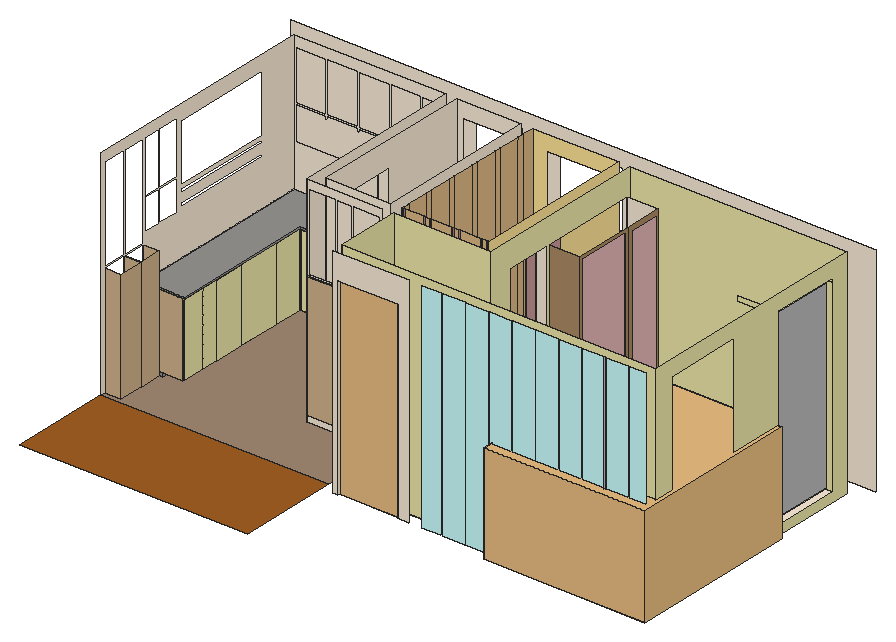
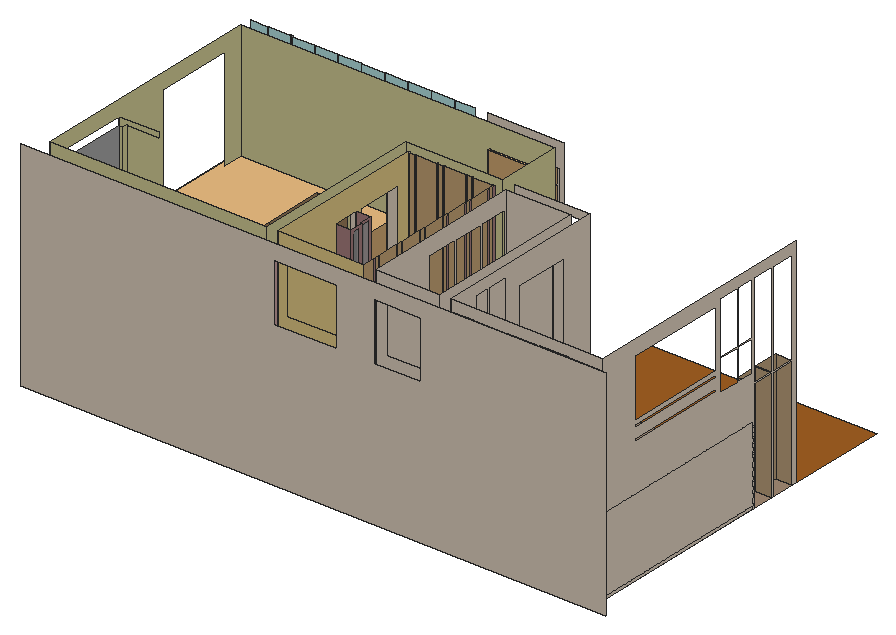
# SketchUp Ruby script. Lengths in inches.
U = 1.inch
M = Sketchup.active_model
def pt(a) = Geom::Point3d.new(a.map { |v| v * U })
def face(e, loops, mat)
  f = e.add_face(loops[0].map { |a| pt(a) })
  loops[1..].each { |l| e.add_face(l.map { |a| pt(a) }).erase! }
  f.material = f.back_material = mat if mat
  f
end
# faces: each face lists its corners as indices into pts; further lists are holes
def faces(e, pts, list, mat = nil) = list.each { |f| face(e, (f[0].is_a?(Array) ? f : [f]).map { |l| l.map { |i| pts[i] } }, mat) }
# xy, xz, yz: faces in a plane at the given z, y or x. An outline is a flat list of corners, or four numbers for a rectangle; further outlines are holes
def ring(l) = l.size == 4 ? [[l[0], l[1]], [l[2], l[1]], [l[2], l[3]], [l[0], l[3]]] : l.each_slice(2).to_a
def flat(e, list, mat, &to3) = list.each { |f| face(e, (f[0].is_a?(Array) ? f : [f]).map { |l| ring(l).map { |u, v| to3.(u, v) } }, mat) }
def xy(e, z, list, mat = nil) = flat(e, list, mat) { |x, y| [x, y, z] }
def xz(e, y, list, mat = nil) = flat(e, list, mat) { |x, z| [x, y, z] }
def yz(e, x, list, mat = nil) = flat(e, list, mat) { |y, z| [x, y, z] }
def lines(e, pts, list) = list.each { |a, b| e.add_line(pt(pts[a]), pt(pts[b])) }
# prism: a flat outline (further loops are holes) pulled along v
def prism(e, loops, v, mat = nil)
  f = face(e, loops, mat); d = Geom::Vector3d.new(v.map { |x| x * U })
  f.pushpull(f.normal.samedirection?(d) ? d.length : -d.length)
end
def box(e, o, s, mat = nil) = prism(e, [[o, [o[0] + s[0], o[1], o[2]], [o[0] + s[0], o[1] + s[1], o[2]], [o[0], o[1] + s[1], o[2]]]], [0, 0, s[2]], mat)
def at(x, y, z, deg = 0) = Geom::Transformation.translation(pt([x, y, z])) * Geom::Transformation.rotation(ORIGIN, Z_AXIS, deg.degrees)
def axes(o, x, y, z) = Geom::Transformation.new([*x, 0, *y, 0, *z, 0, *pt(o).to_a, 1])
def part(name) = M.definitions.add(name)
# library, detail: a bought-in or finely detailed component or shape, given as its bounding box
def library(name, o, s) = part(name).tap { |d| box(d.entities, o, s) }
def detail(e, o, s) = box(e.add_group.entities, o, s)
def put(e, d, t, mat = nil) = e.add_instance(d, t).tap { |i| i.material = mat if mat }
def group(e, t, mat = nil) = e.add_group.tap { |g| g.transformation = t; g.material = mat if mat }.entities
root = M.entities
M.materials.add("Maquette Wood B01 12cm").color = [172, 139, 100]
M.materials.add("Plywood A 50cm\#1").color = [191, 159, 129]
M.materials.add("[0028_AntiqueWhite]").color = [250, 235, 215]
M.materials.add("[0035_Tan]").color = [210, 180, 140]
M.materials.add("[0048_PaleGoldenrod]").color = [238, 232, 170]
M.materials.add("[0119_RosyBrown]").color = [188, 143, 143]
M.materials.add("[0132_LightGray]").color = [169, 169, 169]
M.materials.add("[0134_DimGray]").color = [105, 105, 105]
M.materials.add("[Color D02]").color = [255, 229, 153]
M.materials.add("[Color H01]").color = [204, 255, 255]
M.materials.add("[Color M02]").color = [198, 198, 198]
M.materials.add("[Granite Light Gray]").color = [149, 148, 144]
M.materials.add("[Metal Panel]").color = [255, 255, 255]
M.materials.add("[Mirror 01]").color = [185, 185, 185]
M.materials.add("[Stone Marble]").color = [143, 138, 136]
M.materials.add("[Textile Leaves Green]").color = [226, 183, 181]
M.materials.add("[Tile Ceramic Natural]").color = [255, 255, 255]
M.materials.add("[Translucent Resin Crush Gray]").color = [184, 184, 184]
M.materials["[Translucent Resin Crush Gray]"].alpha = 0.8
M.materials.add("[Travertine Small Tile]").color = [161, 138, 116]
M.materials.add("[Wallpaper Dog Bone]").color = [213, 224, 224]
M.materials.add("[Wallpaper Stripe]").color = [222, 185, 133]
M.materials.add("[Wood Square Tile 02]").color = [160, 95, 34]
M.materials.add("[Wood Veneer 02]").color = [190, 128, 91]
c1 = library("1000x2100 L\#1",[0,0,0],[39.37,8.78,82.68])
c2 = library("Professional+bed",[-16.99,-10.3,0],[85.22,83.04,36.09])
xy(root,0,[[141,369,142.02,369,142.02,369.25,152.78,369.25,152.78,369,153.14,369,153.14,369.25,156.2,369.25,156.2,369,156.7,369,156.7,369.25,168.7,369.25,168.7,369,169.1,369,169.1,369.25,172.1,369.25,172.1,369,172.49,369,172.49,369.25,184.47,369.25,184.47,369,185,369,185,369.25,188,369.25,188,369,189,369,189,375.81,195,375.81,195,401.3125,189,401.3125,189,459,141.1875,459,141.1875,452.4,141,452.4,141,452,141.1875,452,141.1875,449,141,449,141,448.6,141.1875,448.6,141.1875,436.6,141,436.6,141,436.19,141.1875,436.19,141.1875,433.18,141,433.18,141,432.8,141.1875,432.8,141.1875,420.8,141,420.8,141,420.4,141.1875,420.4,141.1875,417.42,141,417.42,141,417,141.1875,417,141.1875,405,141,405,141,404.63,141.1875,404.63,141.1875,401.6,141,401.6,141,401.2,141.1875,401.2,141.1875,389.21,141,389.21,141,388.8,141.1875,388.8,141.1875,385.8,141,385.8,141,385.37,141.1875,385.37,141.1875,373.43,141,373.43,141,373,141.1875,373,141.1875,370,141,370]],"[Metal Panel]")
xy(root,1.45,[[211.3125,404.13,212.3125,434.43]],"[Textile Leaves Green]")
xy(root,1.75,[[9,355.19,9,459,93,459,93,435.69,30.85,435.69,30.85,355.19]],"[0028_AntiqueWhite]")
xy(root,2.25,[[30.85,355.69,31.65,367.69],[30.85,368.19,31.65,376.82],[30.85,377.32,31.65,394.32],[30.85,394.82,31.65,418.32],[30.85,418.82,31.65,434.19],
  [32.35,434.89,44.35,435.69],[44.85,434.89,56.85,435.69],[57.35,434.89,69.35,435.69],[69.85,434.89,81.85,435.69],[82.35,434.89,92.5,435.69]],"[0028_AntiqueWhite]")
xy(root,2.6,[[212.3125,438.47,213,454.22]],"[Textile Leaves Green]")
xy(root,4,[[109.5,361.5625,110.04,361.9375],[110.125,361.5625,110.67,361.9375],[110.75,361.5625,111.3,361.9375],[111.38,361.5625,111.92,361.9375],[112.01,361.5625,112.55,361.9375],
  [112.63,361.5625,113.18,361.9375],[113.26,361.5625,113.8,361.9375],[113.89,361.5625,114.43,361.9375],[114.51,361.5625,115.06,361.9375],[115.14,361.5625,115.68,361.9375],
  [115.76,361.5625,116.31,361.9375],[116.39,361.5625,116.93,361.9375],[117.02,361.5625,117.5625,361.9375],[117.64,361.5625,118.1875,361.9375],[109.5,361.9375,118.1875,363]],"[0028_AntiqueWhite]")
xy(root,4,[[94,361.9375,109,363]],"[0035_Tan]")
xy(root,4,[[118.6875,361.9375,133.6875,363]],"[0048_PaleGoldenrod]")
xy(root,5.3125,[[311,410.9375,315,449.0625]],"[0028_AntiqueWhite]")
xy(root,8.01,[[311,413.64,313.125,446.36]],"[0048_PaleGoldenrod]")
xy(root,12.53,[[181,404.5,181,411.4375,180.4375,411.4375,180.4375,418.8125,189,418.8125,189,404.5]],"[0028_AntiqueWhite]")
xy(root,42,[[30.85,355.69,31.65,367.69],[30.85,368.19,31.65,376.82],[30.85,377.32,31.65,394.32],[30.85,394.82,31.65,418.32],[30.85,418.82,31.65,434.19],
  [32.35,434.89,44.35,435.69],[44.85,434.89,56.85,435.69],[57.35,434.89,69.35,435.69],[69.85,434.89,81.85,435.69],[82.35,434.89,92.5,435.69]],"[0048_PaleGoldenrod]")
xy(root,42.5,[[9,355.19,9,459,93,459,93,434.63,31.91,434.63,31.91,355.19]],"[0028_AntiqueWhite]")
xy(root,43.4375,[[9,355.19,31.91,355.19,31.91,434.63,93,434.63,93,459,9,459]],"[Granite Light Gray]")
xy(root,49.0625,[[99,442.16,134.6875,459]],"[0028_AntiqueWhite]")
xy(root,49.5625,[[101.3125,442.99,117.71,458.18],[118.61,442.99,123.11,458.18]],"[0132_LightGray]")
xy(root,49.6875,[[123.21,442.99,132.0625,446.6]],"[0132_LightGray]")
xy(root,49.75,[[123.21,446.7,132.0625,449.7],[123.21,449.8,132.0625,452.8],[123.21,452.9,132.0625,455.9]],"[0132_LightGray]")
xy(root,49.8125,[[123.21,456,132.0625,458.18]],"[0132_LightGray]")
xy(root,49.875,[[123.11,442.99,123.21,442.99,123.21,446.6,132.0625,446.6,132.0625,446.7,123.21,446.7,123.21,449.7,132.0625,449.7,132.0625,449.8,123.21,449.8,123.21,452.8,132.0625,452.8,132.0625,452.9,123.21,452.9,123.21,455.9,132.0625,455.9,132.0625,456,123.21,456,123.21,458.18,123.11,458.18]],"[0132_LightGray]")
xy(root,49.875,[[[99,442.16,118.61,442.16,118.61,458.18,132.0625,458.18,132.0625,442.99,118.61,442.99,118.61,442.16,134.6875,442.16,134.6875,459,99,459],[101.3125,442.99,117.71,458.18]]],"[Stone Marble]")
xz(root,321,[[141,0,144,0,144,106,177,106,177,0,183,0,183,120,141,120]],"[0028_AntiqueWhite]")
xz(root,321,[[190.25,0,201,120],[201.9,0,213.9,120],[214.8,0,226.8,120],[227.7,0,239.7,120],[240.625,0,252.65,120],
  [253.5,0,265.51,120],[266.47,0,278.4,120],[279.3,0,291.36,120],[292.2,0,304.2,120],[305.01,0,314.1875,120]],"[Color H01]")
xz(root,327,[[141,0,141,120,315,120,315,0,177,0,177,106,144,106,144,0]],"[0048_PaleGoldenrod]")
xz(root,328.1875,[[9,0,18.125,61.75]],"[0035_Tan]")
xz(root,341.8125,[[9,0,18.125,61.75]],"[0035_Tan]")
xz(root,342.3125,[[9,0,18.125,61.75]],"[0035_Tan]")
xz(root,354.625,[[9,0,18.125,61.75]],"[0035_Tan]")
xz(root,355.19,[[9,42.5,31.91,43.4375]],"[Granite Light Gray]")
xz(root,355.69,[[30.85,2.25,31.65,42]],"[0048_PaleGoldenrod]")
xz(root,361.5625,[[109.5,4,110.04,72.59],[110.125,4,110.67,72.59],[110.75,4,111.3,72.59],[111.38,4,111.92,72.59],[112.01,4,112.55,72.59],
  [112.63,4,113.18,72.59],[113.26,4,113.8,72.59],[113.89,4,114.43,72.59],[114.51,4,115.06,72.59],[115.14,4,115.68,72.59],
  [115.76,4,116.31,72.59],[116.39,4,116.93,72.59],[117.02,4,117.5625,72.59],[117.64,4,118.1875,72.59]],"[Wallpaper Dog Bone]")
xz(root,361.9375,[[109.5,4,110.04,72.59],[110.125,4,110.67,72.59],[110.75,4,111.3,72.59],[111.38,4,111.92,72.59],[112.01,4,112.55,72.59],
  [112.63,4,113.18,72.59],[113.26,4,113.8,72.59],[113.89,4,114.43,72.59],[114.51,4,115.06,72.59],[115.14,4,115.68,72.59],
  [115.76,4,116.31,72.59],[116.39,4,116.93,72.59],[117.02,4,117.5625,72.59],[117.64,4,118.1875,72.59]],"[0028_AntiqueWhite]")
xz(root,361.9375,[[94,4,109,72.59]],"[0035_Tan]")
xz(root,361.9375,[[118.6875,4,133.6875,72.59]],"[0048_PaleGoldenrod]")
xz(root,361.9375,[[110.04,4,110.125,72.59],[110.67,4,110.75,72.59],[111.3,4,111.38,72.59],[111.92,4,112.01,72.59],[112.55,4,112.63,72.59],
  [113.18,4,113.26,72.59],[113.8,4,113.89,72.59],[114.43,4,114.51,72.59],[115.06,4,115.14,72.59],[115.68,4,115.76,72.59],
  [116.31,4,116.39,72.59],[116.93,4,117.02,72.59],[117.5625,4,117.64,72.59]],"[Wood Veneer 02]")
xz(root,363,[[[93,0,134.6875,120],[94,4,109,72.59],[118.6875,4,133.6875,72.59],[94,73.1875,109,115.7],[118.6875,73.1875,133.6875,115.7],[109.5,4,118.1875,72.59],[109.5,73.1875,118.1875,115.7]]],"[0028_AntiqueWhite]")
xz(root,363,[[141,0,195,120]],"[0048_PaleGoldenrod]")
xz(root,367.69,[[30.85,2.25,31.65,42]],"[0048_PaleGoldenrod]")
xz(root,368.19,[[30.85,2.25,31.65,42]],"[0048_PaleGoldenrod]")
xz(root,369,[[99,0,99,120,134.6875,120,134.6875,70.71,129.3125,70.71,129.3125,0]],"[0028_AntiqueWhite]")
xz(root,369,[[141,0,142.02,120],[152.78,0,153.14,120],[156.2,0,156.7,120],[168.7,0,169.1,120],[172.1,0,172.49,120],
  [184.47,0,185,120],[188,0,189,120]],"[0119_RosyBrown]")
xz(root,369.25,[[142.02,0,152.78,120],[153.14,0,156.2,120],[156.7,0,168.7,120],[169.1,0,172.1,120],[172.49,0,184.47,120],
  [185,0,188,120]],"[Wallpaper Stripe]")
xz(root,370,[[141,0,141.1875,120]],"[0119_RosyBrown]")
xz(root,373,[[141,0,141.1875,120]],"[0119_RosyBrown]")
xz(root,373.43,[[141,0,141.1875,120]],"[0119_RosyBrown]")
xz(root,375.81,[[189,0,195,106]],"[0028_AntiqueWhite]")
xz(root,376.82,[[30.85,2.25,31.65,42]],"[0048_PaleGoldenrod]")
xz(root,377.32,[[30.85,2.25,31.65,42]],"[0048_PaleGoldenrod]")
xz(root,381.06,[[93,0,99,106]],"[0028_AntiqueWhite]")
xz(root,385.37,[[141,0,141.1875,120]],"[0119_RosyBrown]")
xz(root,385.5,[[129.3125,0,134.6875,70.71]],"[0035_Tan]")
xz(root,385.8,[[141,0,141.1875,120]],"[0119_RosyBrown]")
xz(root,386,[[129.3125,0,134.6875,70.71]],"[0028_AntiqueWhite]")
xz(root,388.8,[[141,0,141.1875,120]],"[0119_RosyBrown]")
xz(root,389.21,[[141,0,141.1875,120]],"[0119_RosyBrown]")
xz(root,394.32,[[30.85,2.25,31.65,42]],"[0048_PaleGoldenrod]")
xz(root,394.82,[[30.85,2.25,31.65,42]],"[0048_PaleGoldenrod]")
xz(root,401.2,[[141,0,141.1875,120]],"[0119_RosyBrown]")
xz(root,401.3125,[[189,0,195,106]],"[0028_AntiqueWhite]")
xz(root,401.6,[[141,0,141.1875,120]],"[0119_RosyBrown]")
xz(root,402.6875,[[195,0,212.3125,106]],"Maquette Wood B01 12cm")
xz(root,403.5,[[129.3125,0,134.6875,70.71]],"[0035_Tan]")
xz(root,404,[[129.3125,0,134.6875,70.71]],"[0035_Tan]")
xz(root,404.13,[[211.3125,1.45,212.3125,104.55]],"[Textile Leaves Green]")
xz(root,404.5,[[181,12.53,189,106]],"[0119_RosyBrown]")
xz(root,404.63,[[141,0,141.1875,120]],"[0119_RosyBrown]")
xz(root,405,[[141,0,141.1875,120]],"[0119_RosyBrown]")
xz(root,410.9375,[[311,5.3125,315,5.3125,315,111.5,293.125,111.5,293.125,108.8,311,108.8]],"[0048_PaleGoldenrod]")
xz(root,411.4375,[[180.4375,12.53,181,106]],"[0119_RosyBrown]")
xz(root,412.0625,[[93,0,99,106]],"[0028_AntiqueWhite]")
xz(root,413.64,[[311,8.01,313.125,108.8]],"[0048_PaleGoldenrod]")
xz(root,417,[[141,0,141.1875,120]],"[0119_RosyBrown]")
xz(root,417.42,[[141,0,141.1875,120]],"[0119_RosyBrown]")
xz(root,418.32,[[30.85,2.25,31.65,42]],"[0048_PaleGoldenrod]")
xz(root,418.8125,[[180.4375,12.53,189,106]],"[0119_RosyBrown]")
xz(root,418.82,[[30.85,2.25,31.65,42]],"[0048_PaleGoldenrod]")
xz(root,420.4,[[141,0,141.1875,120]],"[0119_RosyBrown]")
xz(root,420.8,[[141,0,141.1875,120]],"[0119_RosyBrown]")
xz(root,422,[[129.3125,0,134.6875,70.71]],"[0035_Tan]")
xz(root,432.8,[[141,0,141.1875,120]],"[0119_RosyBrown]")
xz(root,433.18,[[141,0,141.1875,120]],"[0119_RosyBrown]")
xz(root,434.19,[[30.85,2.25,31.65,42]],"[0048_PaleGoldenrod]")
xz(root,434.43,[[211.3125,1.45,212.3125,104.55]],"[Textile Leaves Green]")
xz(root,434.63,[[31.91,42.5,93,43.4375]],"[Granite Light Gray]")
xz(root,434.89,[[32.35,2.25,44.35,42],[44.85,2.25,56.85,42],[57.35,2.25,69.35,42],[69.85,2.25,81.85,42],[82.35,2.25,92.5,42]],"[0048_PaleGoldenrod]")
xz(root,435.69,[[32.35,2.25,44.35,42],[44.85,2.25,56.85,42],[57.35,2.25,69.35,42],[69.85,2.25,81.85,42],[82.35,2.25,92.5,42]],"[0028_AntiqueWhite]")
xz(root,436.19,[[141,0,141.1875,120]],"[0119_RosyBrown]")
xz(root,436.6,[[141,0,141.1875,120]],"[0119_RosyBrown]")
xz(root,438.47,[[212.3125,2.6,213,103.4]],"[Textile Leaves Green]")
xz(root,442.16,[[99,49.0625,134.6875,49.875]],"[Stone Marble]")
xz(root,442.99,[[101.3125,49.5625,117.71,49.875],[118.61,49.5625,123.11,49.875],[123.21,49.6875,132.0625,49.875]],"[0134_DimGray]")
xz(root,446.36,[[311,8.01,313.125,108.8]],"[0048_PaleGoldenrod]")
xz(root,446.6,[[123.21,49.6875,132.0625,49.875]],"[0134_DimGray]")
xz(root,446.7,[[123.21,49.75,132.0625,49.875]],"[0028_AntiqueWhite]")
xz(root,448.6,[[141,0,141.1875,120]],"[0119_RosyBrown]")
xz(root,449,[[141,0,141.1875,120]],"[0119_RosyBrown]")
xz(root,449.0625,[[311,5.3125,315,108.8]],"[0048_PaleGoldenrod]")
xz(root,449.7,[[123.21,49.75,132.0625,49.875]],"[0134_DimGray]")
xz(root,449.8,[[123.21,49.75,132.0625,49.875]],"[0028_AntiqueWhite]")
xz(root,452,[[141,0,141.1875,120]],"[0119_RosyBrown]")
xz(root,452.4,[[141,0,141.1875,120]],"[0119_RosyBrown]")
xz(root,452.8,[[123.21,49.75,132.0625,49.875]],"[0134_DimGray]")
xz(root,452.9,[[123.21,49.75,132.0625,49.875]],"[0028_AntiqueWhite]")
xz(root,454.22,[[212.3125,2.6,213,103.4]],"[Textile Leaves Green]")
xz(root,455.9,[[123.21,49.75,132.0625,49.875]],"[0134_DimGray]")
xz(root,456,[[123.21,49.8125,132.0625,49.875]],"[0028_AntiqueWhite]")
xz(root,456.8125,[[195,0,212.3125,106]],"[0028_AntiqueWhite]")
xz(root,458.18,[[101.3125,49.5625,117.71,49.875],[118.61,49.5625,123.11,49.875],[123.21,49.8125,132.0625,49.875]],"[0134_DimGray]")
xz(root,459,[[9,0,93,1.75],[99,0,113.74,49.0625],[113.74,0,134.6875,49.0625],[[9,43.4375,93,120],[10,67.4375,10,86.125,27,86.125,27,84.6875,27.5,84.6875,27.5,86.125,44.5,86.125,44.5,84.6875,45,84.6875,45,86.125,62,86.125,62,84.6875,62.5,84.6875,62.5,86.125,79.5,86.125,79.5,84.6875,80,84.6875,80,86.125,92,86.125,92,67.4375],[10,86.6875,27,114.3125],[27.5,86.6875,44.5,114.3125],[45,86.6875,62,114.3125],[62.5,86.6875,79.5,114.3125],[80,86.6875,92,114.3125]],[99,49.0625,134.6875,49.875],
  [[99,49.875,134.6875,120],[102.5,79.6875,128.4375,111.66]]],"[0028_AntiqueWhite]")
xz(root,459,[[195,0,315,120]],"[0048_PaleGoldenrod]")
xz(root,459,[[[141.1875,0,189,120],[148.875,79.6875,183.6875,111.66]]],"[Color D02]")
xz(root,468,[[[0,0,324,120],[148.875,79.6875,183.6875,111.66],[102.5,79.6875,128.4375,111.66]]],"[0028_AntiqueWhite]")
yz(root,9,[[[325.9375,0,328.1875,0,328.1875,61.75,341.8125,61.75,341.8125,0,342.3125,0,342.3125,61.75,354.625,61.75,354.625,0,355.19,0,355.19,43.4375,459,43.4375,459,120,325.9375,120],[380.875,79.6875,437.125,111.66],[328.1875,62.3125,341.8125,114.3125],[342.3125,62.3125,354.625,114.3125],[365.9375,85.02,377.9375,114.3125],[355.875,85.02,365.4375,114.3125],[365.9375,67.4375,377.9375,84.71],[355.875,67.4375,365.4375,84.71],[380.875,76.0625,437.125,77.6875],[380.875,69.2,437.125,70.77]],[355.19,0,459,1.75],[355.19,1.75,459,43.4375]],"[0028_AntiqueWhite]")
yz(root,18.125,[[328.1875,0,341.8125,61.75],[342.3125,0,354.625,61.75]],"[0035_Tan]")
yz(root,30.85,[[355.69,2.25,367.69,42],[368.19,2.25,376.82,42],[377.32,2.25,394.32,42],[394.82,2.25,418.32,42],[418.82,2.25,434.19,42]],"[0028_AntiqueWhite]")
yz(root,31.65,[[355.69,2.25,367.69,42],[368.19,2.25,376.82,42],[377.32,2.25,394.32,42],[394.82,2.25,418.32,42],[418.82,2.25,434.19,42]],"[0048_PaleGoldenrod]")
yz(root,31.91,[[355.19,42.5,434.63,43.4375]],"[Granite Light Gray]")
yz(root,32.35,[[434.89,2.25,435.69,42]],"[0048_PaleGoldenrod]")
yz(root,44.35,[[434.89,2.25,435.69,42]],"[0048_PaleGoldenrod]")
yz(root,44.85,[[434.89,2.25,435.69,42]],"[0048_PaleGoldenrod]")
yz(root,56.85,[[434.89,2.25,435.69,42]],"[0048_PaleGoldenrod]")
yz(root,57.35,[[434.89,2.25,435.69,42]],"[0048_PaleGoldenrod]")
yz(root,69.35,[[434.89,2.25,435.69,42]],"[0048_PaleGoldenrod]")
yz(root,69.85,[[434.89,2.25,435.69,42]],"[0048_PaleGoldenrod]")
yz(root,81.85,[[434.89,2.25,435.69,42]],"[0048_PaleGoldenrod]")
yz(root,82.35,[[434.89,2.25,435.69,42]],"[0048_PaleGoldenrod]")
yz(root,92.5,[[434.89,2.25,435.69,42]],"[0048_PaleGoldenrod]")
yz(root,93,[[[363,0,363,120,459,120,459,43.4375,434.63,43.4375,434.63,42.5,435.69,42.5,435.69,1.75,449.82,1.75,449.82,0,412.0625,0,412.0625,106,381.06,106,381.06,0],[421,67.4375,441.5625,67.4375,441.5625,86.125,433.5,86.125,433.5,84.6875,433,84.6875,433,86.125,421,86.125],[421,86.6875,433,114.3125],[433.5,86.6875,441.5625,114.3125]],[449.82,0,459,1.75]],"[0028_AntiqueWhite]")
yz(root,94,[[361.9375,4,363,72.59]],"[0035_Tan]")
yz(root,99,[[369,0,381.06,0,381.06,106,412.0625,106,412.0625,0,459,0,459,120,369,120]],"[0028_AntiqueWhite]")
yz(root,101.3125,[[442.99,49.5625,458.18,49.875]],"[0134_DimGray]")
yz(root,109,[[361.9375,4,363,72.59]],"[0035_Tan]")
yz(root,109.5,[[361.5625,4,361.9375,72.59]],"[Wallpaper Dog Bone]")
yz(root,109.5,[[361.9375,4,363,72.59]],"[Wood Veneer 02]")
yz(root,110.04,[[361.5625,4,361.9375,72.59]],"[Wallpaper Dog Bone]")
yz(root,110.125,[[361.5625,4,361.9375,72.59]],"[Wallpaper Dog Bone]")
yz(root,110.67,[[361.5625,4,361.9375,72.59]],"[Wallpaper Dog Bone]")
yz(root,110.75,[[361.5625,4,361.9375,72.59]],"[Wallpaper Dog Bone]")
yz(root,111.3,[[361.5625,4,361.9375,72.59]],"[Wallpaper Dog Bone]")
yz(root,111.38,[[361.5625,4,361.9375,72.59]],"[Wallpaper Dog Bone]")
yz(root,111.92,[[361.5625,4,361.9375,72.59]],"[Wallpaper Dog Bone]")
yz(root,112.01,[[361.5625,4,361.9375,72.59]],"[Wallpaper Dog Bone]")
yz(root,112.55,[[361.5625,4,361.9375,72.59]],"[Wallpaper Dog Bone]")
yz(root,112.63,[[361.5625,4,361.9375,72.59]],"[Wallpaper Dog Bone]")
yz(root,113.18,[[361.5625,4,361.9375,72.59]],"[Wallpaper Dog Bone]")
yz(root,113.26,[[361.5625,4,361.9375,72.59]],"[Wallpaper Dog Bone]")
yz(root,113.8,[[361.5625,4,361.9375,72.59]],"[Wallpaper Dog Bone]")
yz(root,113.89,[[361.5625,4,361.9375,72.59]],"[Wallpaper Dog Bone]")
yz(root,114.43,[[361.5625,4,361.9375,72.59]],"[Wallpaper Dog Bone]")
yz(root,114.51,[[361.5625,4,361.9375,72.59]],"[Wallpaper Dog Bone]")
yz(root,115.06,[[361.5625,4,361.9375,72.59]],"[Wallpaper Dog Bone]")
yz(root,115.14,[[361.5625,4,361.9375,72.59]],"[Wallpaper Dog Bone]")
yz(root,115.68,[[361.5625,4,361.9375,72.59]],"[Wallpaper Dog Bone]")
yz(root,115.76,[[361.5625,4,361.9375,72.59]],"[Wallpaper Dog Bone]")
yz(root,116.31,[[361.5625,4,361.9375,72.59]],"[Wallpaper Dog Bone]")
yz(root,116.39,[[361.5625,4,361.9375,72.59]],"[Wallpaper Dog Bone]")
yz(root,116.93,[[361.5625,4,361.9375,72.59]],"[Wallpaper Dog Bone]")
yz(root,117.02,[[361.5625,4,361.9375,72.59]],"[Wallpaper Dog Bone]")
yz(root,117.5625,[[361.5625,4,361.9375,72.59]],"[Wallpaper Dog Bone]")
yz(root,117.64,[[361.5625,4,361.9375,72.59]],"[Wallpaper Dog Bone]")
yz(root,117.71,[[442.99,49.5625,458.18,49.875]],"[0134_DimGray]")
yz(root,118.1875,[[361.5625,4,361.9375,72.59]],"[Wallpaper Dog Bone]")
yz(root,118.1875,[[361.9375,4,363,72.59]],"[Wood Veneer 02]")
yz(root,118.61,[[442.99,49.5625,458.18,49.875]],"[0028_AntiqueWhite]")
yz(root,118.6875,[[361.9375,4,363,72.59]],"[0048_PaleGoldenrod]")
yz(root,123.11,[[442.99,49.5625,458.18,49.875]],"[0028_AntiqueWhite]")
yz(root,123.21,[[442.99,49.6875,446.6,49.875],[446.7,49.75,449.7,49.875],[449.8,49.75,452.8,49.875],[452.9,49.75,455.9,49.875],[456,49.8125,458.18,49.875]],"[0028_AntiqueWhite]")
yz(root,129.3125,[[369,0,385.5,70.71],[386,0,403.5,70.71],[404,0,422,70.71]],"[0035_Tan]")
yz(root,132.0625,[[442.99,49.6875,446.6,49.875],[446.7,49.75,449.7,49.875],[449.8,49.75,452.8,49.875],[452.9,49.75,455.9,49.875],[456,49.8125,458.18,49.875]],"[0028_AntiqueWhite]")
yz(root,133.6875,[[361.9375,4,363,72.59]],"[0048_PaleGoldenrod]")
yz(root,134.6875,[[[385.5,0,385.5,70.71,369,70.71,369,120,459,120,459,49.875,442.16,49.875,442.16,49.0625,459,49.0625,459,0,422,0,422,70.71,404,70.71,404,0,403.5,0,403.5,70.71,386,70.71,386,0],[404,71.3125,422,110.4375],[386,71.3125,403.5,110.4375],[369.5,71.3125,385.5,110.4375]]],"[0028_AntiqueWhite]")
yz(root,141,[[327,0,363,120]],"[0048_PaleGoldenrod]")
yz(root,141,[[369,0,370,120],[373,0,373.43,120],[385.37,0,385.8,120],[388.8,0,389.21,120],[401.2,0,401.6,120],
  [404.63,0,405,120],[417,0,417.42,120],[420.4,0,420.8,120],[432.8,0,433.18,120],[436.19,0,436.6,120],
  [448.6,0,449,120],[452,0,452.4,120]],"[0119_RosyBrown]")
yz(root,141.1875,[[370,0,373,120],[373.43,0,385.37,120],[385.8,0,388.8,120],[389.21,0,401.2,120],[401.6,0,404.63,120],
  [405,0,417,120],[417.42,0,420.4,120],[420.8,0,432.8,120],[433.18,0,436.19,120],[436.6,0,448.6,120],
  [449,0,452,120],[452.4,0,459,120]],"[Wallpaper Stripe]")
yz(root,142.02,[[369,0,369.25,120]],"[0119_RosyBrown]")
yz(root,144,[[321,0,327,106]],"[0028_AntiqueWhite]")
yz(root,152.78,[[369,0,369.25,120]],"[0119_RosyBrown]")
yz(root,153.14,[[369,0,369.25,120]],"[0119_RosyBrown]")
yz(root,156.2,[[369,0,369.25,120]],"[0119_RosyBrown]")
yz(root,156.7,[[369,0,369.25,120]],"[0119_RosyBrown]")
yz(root,168.7,[[369,0,369.25,120]],"[0119_RosyBrown]")
yz(root,169.1,[[369,0,369.25,120]],"[0119_RosyBrown]")
yz(root,172.1,[[369,0,369.25,120]],"[0119_RosyBrown]")
yz(root,172.49,[[369,0,369.25,120]],"[0119_RosyBrown]")
yz(root,177,[[321,0,327,106]],"[0028_AntiqueWhite]")
yz(root,180.4375,[[[411.4375,12.53,418.8125,106],[413.41,14.51,416.84,104.02]]],"[0119_RosyBrown]")
yz(root,180.4375,[[413.41,14.51,416.84,104.02]],"[Translucent Resin Crush Gray]")
yz(root,181,[[[404.5,12.53,411.4375,106],[405.99,14.02,409.94,104.51]]],"[0119_RosyBrown]")
yz(root,181,[[405.99,14.02,409.94,104.51]],"[Translucent Resin Crush Gray]")
yz(root,184.47,[[369,0,369.25,120]],"[0119_RosyBrown]")
yz(root,185,[[369,0,369.25,120]],"[0119_RosyBrown]")
yz(root,188,[[369,0,369.25,120]],"[0028_AntiqueWhite]")
yz(root,189,[[[369,0,369,120,459,120,459,0,401.3125,0,401.3125,106,375.81,106,375.81,0],[404.5,12.53,418.8125,106]]],"[Color D02]")
yz(root,195,[[363,0,375.81,0,375.81,106,401.3125,106,401.3125,0,402.6875,0,402.6875,106,456.8125,106,456.8125,0,459,0,459,120,363,120]],"[0048_PaleGoldenrod]")
yz(root,211.3125,[[404.13,1.45,434.43,104.55]],"[Textile Leaves Green]")
yz(root,212.3125,[[[402.6875,0,435.875,106],[404.13,1.45,434.43,104.55]],[[435.875,0,456.8125,106],[438.47,2.6,454.22,103.4]]],"Maquette Wood B01 12cm")
yz(root,213,[[438.47,2.6,454.22,103.4]],"[Textile Leaves Green]")
yz(root,291.36,[[320.4375,0,321,120]],"[Color M02]")
yz(root,292.2,[[320.4375,0,321,120]],"[Color M02]")
yz(root,311,[[410.9375,5.3125,410.9375,108.8,413.64,108.8,413.64,8.01,446.36,8.01,446.36,108.8,449.0625,108.8,449.0625,5.3125]],"[0048_PaleGoldenrod]")
yz(root,313.125,[[413.64,8.01,446.36,108.8]],"[Mirror 01]")
yz(root,315,[[[327,0,459,120],[410.9375,5.3125,449.0625,111.5],[337.5625,52.5,381.0625,111.5]]],"[0048_PaleGoldenrod]")
p = [[135,363,0],[134.6875,363,0],[93,412.0625,0],[93,381.06,0],[18.4375,355.19,0],[9,355.19,0],
  [18.4375,449.82,0],[93,449.82,0]]
lines(root,p,[[0,1],[2,3],[4,5],[6,4],[7,6]])
put(root,c1,axes([144,321.98,0],[0.8382,0,0],[0,0.74,0],[0,0,1.29492]))
put(root,c2,axes([239.73,391.81,0],[0,-1.11,0],[1.07222,0,0],[0,0,1.5318]))
g1 = group(root,at(9,270,0),"[Wood Square Tile 02]")
xy(g1,0,[[0,55.9375,125.6875,55.9375,125.6875,93,84,93,84,189,0,189]],"[Travertine Small Tile]")
xy(g1,0,[[0,0,125.6875,55.9375]],"[Wood Square Tile 02]")
g2 = group(root,at(141,327,0),"[0028_AntiqueWhite]")
xy(g2,0,[[0,0,174,0,174,132,54,132,54,36,0,36]],"[Tile Ceramic Natural]")
g3 = group(root,at(9,355.19,0),"[0028_AntiqueWhite]")
xy(g3,1.75,[[0,0,10.8125,0,10.8125,94.625,84,94.625,84,103.81,0,103.81]])
xz(g3,0,[[0,0,10.8125,1.75]],"[Granite Light Gray]")
xz(g3,94.625,[[10.8125,0,84,1.75]])
yz(g3,10.8125,[[0,0,94.625,1.75]],"[Granite Light Gray]")
g4 = group(root,at(9,355.19,1.75),"[0028_AntiqueWhite]")
xy(g4,40.75,[[0,0,21.85,0,21.85,80.5,84,80.5,84,103.81,0,103.81]],"[0035_Tan]")
xz(g4,0,[[0,0,21.85,40.75]],"[0035_Tan]")
xz(g4,80.5,[[21.85,0,84,40.75]],"[0035_Tan]")
yz(g4,21.85,[[0,0,80.5,40.75]],"[0035_Tan]")
g5 = group(root,at(93,369,0),"[0028_AntiqueWhite]")
xy(g5,0,[[6,0,41.6875,0,41.6875,90,6,90,6,43.0625,0,43.0625,0,12.06,6,12.06]],"[Travertine Small Tile]")
g6 = group(root,at(99,427.6875,0),"[0028_AntiqueWhite]")
xy(g6,0,[[14.74,15.625,35.6875,31.3125]])
xy(g6,49.0625,[[0,15.4375,14.74,15.4375,14.74,15.625,35.6875,15.625,35.6875,31.3125,0,31.3125]])
xz(g6,15.4375,[[0,0,14.74,49.0625]],"Plywood A 50cm\#1")
xz(g6,15.625,[[14.74,0,35.6875,49.0625]],"Plywood A 50cm\#1")
xz(g6,31.3125,[[14.74,0,35.6875,49.0625]])
yz(g6,14.74,[[15.4375,0,15.625,49.0625]],"Plywood A 50cm\#1")
yz(g6,35.6875,[[15.625,0,31.3125,49.0625]])
